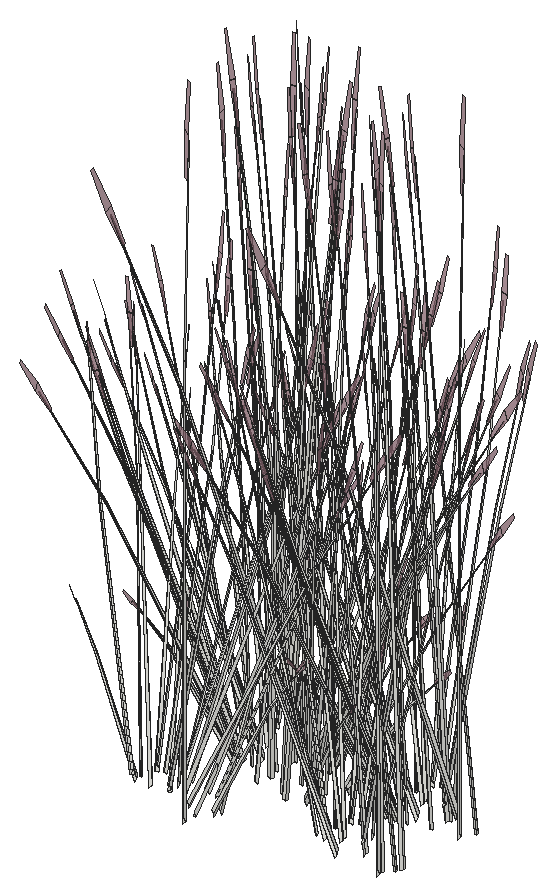
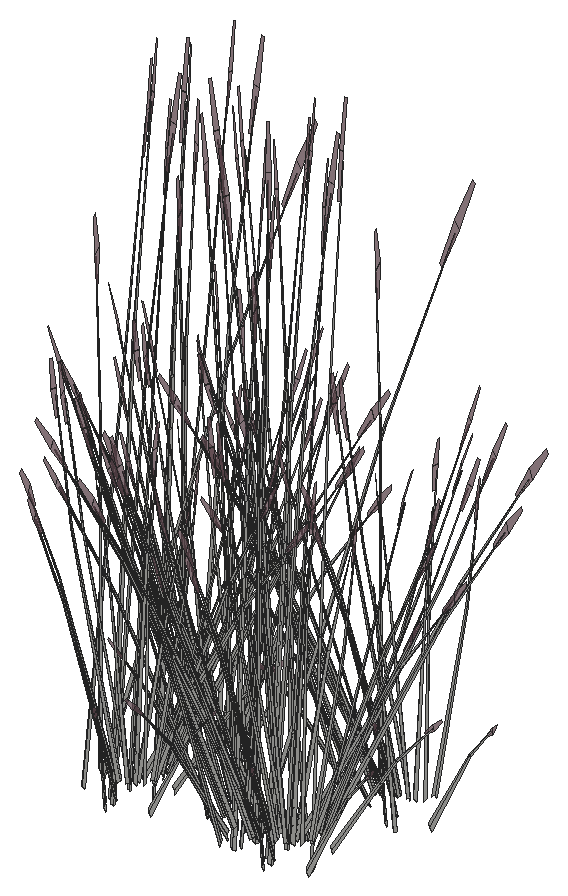
# SketchUp Ruby script. Lengths in inches.
U = 1.inch
M = Sketchup.active_model
def pt(a) = Geom::Point3d.new(a.map { |v| v * U })
def face(e, loops, mat)
  f = e.add_face(loops[0].map { |a| pt(a) })
  loops[1..].each { |l| e.add_face(l.map { |a| pt(a) }).erase! }
  f.material = f.back_material = mat if mat
  f
end
# faces: each face lists its corners as indices into pts; further lists are holes
def faces(e, pts, list, mat = nil) = list.each { |f| face(e, (f[0].is_a?(Array) ? f : [f]).map { |l| l.map { |i| pts[i] } }, mat) }
# xy, xz, yz: faces in a plane at the given z, y or x. An outline is a flat list of corners, or four numbers for a rectangle; further outlines are holes
def ring(l) = l.size == 4 ? [[l[0], l[1]], [l[2], l[1]], [l[2], l[3]], [l[0], l[3]]] : l.each_slice(2).to_a
def flat(e, list, mat, &to3) = list.each { |f| face(e, (f[0].is_a?(Array) ? f : [f]).map { |l| ring(l).map { |u, v| to3.(u, v) } }, mat) }
def xy(e, z, list, mat = nil) = flat(e, list, mat) { |x, y| [x, y, z] }
def xz(e, y, list, mat = nil) = flat(e, list, mat) { |x, z| [x, y, z] }
def yz(e, x, list, mat = nil) = flat(e, list, mat) { |y, z| [x, y, z] }
def lines(e, pts, list) = list.each { |a, b| e.add_line(pt(pts[a]), pt(pts[b])) }
# prism: a flat outline (further loops are holes) pulled along v
def prism(e, loops, v, mat = nil)
  f = face(e, loops, mat); d = Geom::Vector3d.new(v.map { |x| x * U })
  f.pushpull(f.normal.samedirection?(d) ? d.length : -d.length)
end
def box(e, o, s, mat = nil) = prism(e, [[o, [o[0] + s[0], o[1], o[2]], [o[0] + s[0], o[1] + s[1], o[2]], [o[0], o[1] + s[1], o[2]]]], [0, 0, s[2]], mat)
def at(x, y, z, deg = 0) = Geom::Transformation.translation(pt([x, y, z])) * Geom::Transformation.rotation(ORIGIN, Z_AXIS, deg.degrees)
def axes(o, x, y, z) = Geom::Transformation.new([*x, 0, *y, 0, *z, 0, *pt(o).to_a, 1])
def part(name) = M.definitions.add(name)
# library, detail: a bought-in or finely detailed component or shape, given as its bounding box
def library(name, o, s) = part(name).tap { |d| box(d.entities, o, s) }
def detail(e, o, s) = box(e.add_group.entities, o, s)
def put(e, d, t, mat = nil) = e.add_instance(d, t).tap { |i| i.material = mat if mat }
def group(e, t, mat = nil) = e.add_group.tap { |g| g.transformation = t; g.material = mat if mat }.entities
root = M.entities
M.materials.add("LightPink_Translucent").color = [144, 107, 117]
M.materials["LightPink_Translucent"].alpha = 0.75
c1 = part("blade")
p = [[2.15,0.21,22],[0,0.17,0],[0.09,0.45,0],[2.18,0.31,22],[2.29,0.31,22],[0.38,0.45,0],
  [2.48,0.24,33],[2.49,0.24,33],[2.48,0.22,33]]
faces(c1.entities,p,[[0,1,2,3],[4,5,2,3],[6,3,4,7],[8,0,3,6]])
c2 = part("seeds")
p = [[0.3,-0.1,1.38],[-0.01,-0.03,1.59],[-0.01,-0.03,0.03],[0.14,-0.07,-0.07],[0.29,-0.03,3],[0.15,0.01,3.11]]
faces(c2.entities,p,[[0,1,2,3],[1,0,4,5]],"LightPink_Translucent")
c3 = part("blade with seeds")
put(c3.entities,c1,at(0,0,0))
put(c3.entities,c2,axes([2.4,0.25,30.99],[1.5799,-0.05474,1.17369],[-0.12525,1.92788,0.29478],[-0.07173,-0.02425,1.56792]))
put(root,c3,axes([679.34,344.25,512.05],[0.18794,-0.56744,0.14643],[0.68774,0.16058,0.29122],[-0.1188,0.00276,1.33138]))
put(root,c3,axes([677.89,346.63,513.76],[-0.10048,-0.4599,-0.29394],[0.5744,-0.12144,0.37948],[-0.15428,-0.13179,0.72609]))
put(root,c3,axes([661.52,342.6,512.3],[0.27113,-0.25877,0.95334],[0.10699,0.40966,0.70045],[-0.19594,0.07335,0.20998]))
put(root,c3,axes([668.04,342.12,513.76],[0.37017,0.35748,-0.29394],[-0.42268,0.3384,0.37948],[0.21476,0.05149,0.72609]))
put(root,c3,axes([676.6,342.27,512.77],[0.18493,-0.0826,1.46963],[0.06377,0.5767,0.11501],[-0.40056,0.07652,0.52526]))
put(root,c3,axes([662.54,341.48,513.76],[-0.56631,0.0816,-0.29394],[-0.14954,-0.46647,0.37948],[-0.16229,0.12529,0.72609]))
put(root,c3,axes([677.03,344.51,512.06],[0.60889,0.28548,0.4121],[-0.36394,0.51192,0],[-0.13868,-0.06502,1.30728]))
put(root,c3,axes([665.35,347.1,513.22],[0.24166,0.09837,1.42242],[-0.50011,0.41269,0.11501],[-0.3117,-0.18617,0.60807]))
put(root,c3,axes([676.66,347.3,513.22],[0.24166,0.09837,1.42242],[-0.50011,0.41269,0.11501],[-0.3117,-0.18617,0.60807]))
put(root,c3,axes([675.33,342.59,513.89],[-0.17625,0.51936,-0.42412],[-0.60429,-0.17802,-0.32852],[-0.2433,0.04762,0.81151]))
put(root,c3,axes([666.52,346.81,513.89],[-0.64198,0.13573,-0.42412],[-0.1123,-0.514,-0.32852],[-0.17243,-0.1473,0.81151]))
put(root,c3,axes([666.71,341.2,513.22],[-0.24166,-0.09837,1.42242],[0.50011,-0.41269,0.11501],[0.3117,0.18617,0.60807]))
put(root,c3,axes([679.01,343.25,512.26],[0.70648,-0.03525,0.37133],[0.06389,0.58508,-0.17871],[-0.12647,0.0593,1.19224]))
put(root,c3,axes([677.82,347.01,513.89],[-0.64198,0.13573,-0.42412],[-0.1123,-0.514,-0.32852],[-0.17243,-0.1473,0.81151]))
put(root,c3,axes([670.31,348.03,514.13],[0.33983,-0.45051,-0.58968],[0.59551,0.32017,0.07116],[0.20291,-0.16322,0.83415]))
put(root,c3,axes([670.29,347.82,513.89],[-0.16713,-0.52135,-0.42412],[0.63294,-0.0912,-0.32852],[0.18138,-0.14003,0.81151]))
put(root,c3,axes([667.61,342.32,512.3],[-0.36631,-0.16417,0.95334],[0.47299,-0.16681,0.70045],[0.12758,0.1413,0.20998]))
put(root,c3,axes([663.01,341.53,513.89],[0.16713,0.52135,-0.42412],[-0.63294,0.0912,-0.32852],[-0.18138,0.14003,0.81151]))
put(root,c3,axes([668.1,349.91,512.76],[0.56221,0.23024,1.25546],[-0.55078,0.49601,0.49647],[-0.2467,-0.29398,1.05249]))
put(root,c3,axes([666.72,340.47,512.36],[-0.01777,-0.53759,1.17256],[0.80434,0.13935,0.49647],[-0.19024,0.29416,1.1068]))
put(root,c3,axes([675.31,342.85,513.22],[0.22574,-0.12077,1.42242],[0.19004,0.55807,0.11501],[-0.35439,0.12613,0.60807]))
put(root,c3,axes([666.78,342.55,513.89],[0.64198,-0.13573,-0.42412],[0.1123,0.514,-0.32852],[0.17243,0.1473,0.81151]))
put(root,c3,axes([679.41,350.12,512.76],[0.56221,0.23024,1.25546],[-0.55078,0.49601,0.49647],[-0.2467,-0.29398,1.05249]))
put(root,c3,axes([671.07,346.79,512.3],[-0.2167,0.29065,0.95334],[-0.18626,-0.3905,0.70045],[0.17898,-0.09785,0.20998]))
put(root,c3,axes([667.67,343.07,512.21],[-0.4172,-0.01791,0.872],[0.27552,-0.38032,0.48145],[0.16481,0.13512,0.68401]))
put(root,c3,axes([679.53,344.55,512.06],[0.60889,-0.28548,0.4121],[0.36394,0.51192,0],[-0.13868,0.06502,1.30728]))
put(root,c3,axes([670.76,347.88,513.76],[0.56631,-0.0816,-0.29394],[0.14954,0.46647,0.37948],[0.16229,-0.12529,0.72609]))
put(root,c3,axes([665.25,347.24,513.76],[-0.37017,-0.35748,-0.29394],[0.42268,-0.3384,0.37948],[-0.21476,-0.05149,0.72609]))
put(root,c3,axes([663.4,341.45,513.22],[0.12114,-0.19625,1.42242],[0.50818,0.40613,0.11501],[-0.22925,0.25313,0.60807]))
put(root,c3,axes([674.13,344.81,512.3],[0.27113,-0.25877,0.95334],[0.10699,0.40966,0.70045],[-0.19594,0.07335,0.20998]))
put(root,c3,axes([676.5625,347.44,513.76],[-0.37017,-0.35748,-0.29394],[0.42268,-0.3384,0.37948],[-0.21476,-0.05149,0.72609]))
put(root,c3,axes([666.31,342.15,512.15],[0.01148,-0.18927,1.18691],[0.54864,-0.21141,-0.25526],[0.16937,0.22654,0.50747]))
put(root,c3,axes([675.15,343.6875,513.76],[-0.56631,0.0816,-0.29394],[-0.14954,-0.46647,0.37948],[-0.16229,0.12529,0.72609]))
put(root,c3,axes([663.54,342.56,513.76],[-0.4402,0.30062,-0.29394],[-0.41671,-0.34326,0.37948],[-0.0634,0.1744,0.72609]))
put(root,c3,axes([663.82,343.72,512.3],[-0.01684,-0.3395,0.95334],[0.42072,0.24214,0.70045],[-0.08274,0.16182,0.20998]))
put(root,c3,axes([665.64,347.47,514.13],[-0.65035,-0.01375,-0.58968],[0.04368,-0.5789,0.07116],[-0.27552,-0.06109,0.83415]))
put(root,c3,axes([676.95,347.68,514.13],[-0.65035,-0.01375,-0.58968],[0.04368,-0.5789,0.07116],[-0.27552,-0.06109,0.83415]))
put(root,c3,axes([663.97,342.41,514.15],[0.46573,0.38364,-0.47077],[-0.49199,0.33598,-0.36465],[-0.07086,0.19492,0.90078]))
put(root,c3,axes([665.36,342.79,513.89],[0.63954,0.14313,-0.42412],[-0.21921,0.49074,-0.32852],[0.05864,0.19758,0.81151]))
put(root,c3,axes([665.72,341.77,513.22],[-0.14872,-0.18332,1.42242],[0.6872,-0.15433,0.11501],[0.15531,0.28779,0.60807]))
put(root,c3,axes([665.0625,343.09,513.76],[-0.19614,0.43908,-0.29394],[-0.57222,-0.12807,0.37948],[0.05247,0.17678,0.72609]))
put(root,c3,axes([676.13,343.23,513.22],[0.1625,-0.17544,1.42242],[0.41029,0.47354,0.11501],[-0.28141,0.21565,0.60807]))
put(root,c3,axes([665.43,347.59,513.89],[-0.47241,0.37822,-0.42412],[-0.41372,-0.39954,-0.32852],[-0.24002,-0.05755,0.81151]))
put(root,c3,axes([663.83,342.24,514.43],[-0.01693,0.52814,-0.65454],[-0.71285,-0.03547,0.07899],[-0.07523,0.22375,0.92591]))
put(root,c3,axes([675.62,343.74,513.89],[0.16713,0.52135,-0.42412],[-0.63294,0.0912,-0.32852],[-0.18138,0.14003,0.81151]))
put(root,c3,axes([664.36,348.09,512.3],[0.41536,-0.04086,0.95334],[-0.26347,0.35999,0.70045],[-0.20525,-0.054,0.20998]))
put(root,c3,axes([676.74,347.8,513.89],[-0.47241,0.37822,-0.42412],[-0.41372,-0.39954,-0.32852],[-0.24002,-0.05755,0.81151]))
put(root,c3,axes([664.5,341.86,513.22],[-0.01592,-0.21915,1.42242],[0.69015,0.14538,0.11501],[-0.04269,0.3123,0.60807]))
put(root,c3,axes([679.33,342.6875,512.36],[-0.01777,-0.53759,1.17256],[0.80434,0.13935,0.49647],[-0.19024,0.29416,1.1068]))
put(root,c3,axes([667.3,348.43,512.26],[-0.70648,0.03525,0.37133],[-0.06389,-0.58508,-0.17871],[0.12647,-0.0593,1.19224]))
put(root,c3,axes([665.48,348.85,512.06],[0,0.57097,0.4121],[-0.72788,0,0],[0,-0.13004,1.30728]))
put(root,c3,axes([675.67,348.3,512.3],[0.41536,-0.04086,0.95334],[-0.26347,0.35999,0.70045],[-0.20525,-0.054,0.20998]))
put(root,c3,axes([670.58,348.98,513.89],[0.17625,-0.51936,-0.42412],[0.60429,0.17802,-0.32852],[0.2433,-0.04762,0.81151]))
put(root,c3,axes([664.84,348,513.22],[0.26985,-0.01293,1.42242],[-0.17902,0.56047,0.11501],[-0.38456,-0.03467,0.60807]))
put(root,c3,axes([665.125,342.69,514.13],[0.31051,0.46426,-0.58968],[-0.63919,0.25873,0.07116],[0.07261,0.22432,0.83415]))
put(root,c3,axes([676.78,349.06,512.06],[0,0.57097,0.4121],[-0.72788,0,0],[0,-0.13004,1.30728]))
put(root,c3,axes([663.33,343.42,512.15],[0.2053,-0.09007,1.18691],[0.50689,0.27159,-0.25526],[-0.15087,0.235,0.50747]))
put(root,c3,axes([676.15,348.2,513.22],[0.26985,-0.01293,1.42242],[-0.17902,0.56047,0.11501],[-0.38456,-0.03467,0.60807]))
put(root,c3,axes([667.13,349.14,512.26],[-0.31565,0.51449,0.37133],[-0.65588,-0.24761,-0.17871],[0,-0.1186,1.19224]))
put(root,c3,axes([669.28,347.16,512.06],[-0.60889,-0.28548,0.4121],[0.36394,-0.51192,0],[0.13868,0.06502,1.30728]))
put(root,c3,axes([670.47,349.17,514.13],[0.57168,-0.25217,-0.58968],[0.3186,0.51908,0.07116],[0.27622,-0.05897,0.83415]))
put(root,c3,axes([678.44,349.34,512.26],[-0.31565,0.51449,0.37133],[-0.65588,-0.24761,-0.17871],[0,-0.1186,1.19224]))
put(root,c3,axes([676.01,343.66,513.22],[0.12114,-0.19625,1.42242],[0.50818,0.40613,0.11501],[-0.22925,0.25313,0.60807]))
put(root,c3,axes([666.97,347.42,512.05],[-0.18794,0.56744,0.14643],[-0.68774,-0.16058,0.29122],[0.1188,-0.00276,1.33138]))
put(root,c3,axes([663.59,342.98,512.79],[0.01429,-0.29475,1.28107],[0.64291,0.15569,0.17703],[-0.0557,0.31414,0.60492]))
put(root,c3,axes([676.15,344.77,513.76],[-0.4402,0.30062,-0.29394],[-0.41671,-0.34326,0.37948],[-0.0634,0.1744,0.72609]))
put(root,c3,axes([676.43,345.9375,512.3],[-0.01684,-0.3395,0.95334],[0.42072,0.24214,0.70045],[-0.08274,0.16182,0.20998]))
put(root,c3,axes([668.14,348.1875,512.26],[-0.39083,-0.47924,0.37133],[0.59199,-0.33747,-0.17871],[0.12647,0.0593,1.19224]))
put(root,c3,axes([666.9,350.35,512.05],[0.6991,-0.15154,0.14643],[0.17263,0.56398,0.29122],[-0.06235,-0.08217,1.33138]))
put(root,c3,axes([670.95,349.22,513.76],[0.54068,0.15928,-0.29394],[-0.1577,0.46469,0.37948],[0.21769,-0.04261,0.72609]))
put(root,c3,axes([676.59,344.625,514.15],[0.46573,0.38364,-0.47077],[-0.49199,0.33598,-0.36465],[-0.07086,0.19492,0.90078]))
put(root,c3,axes([664.6,348.48,513.76],[-0.54068,-0.15928,-0.29394],[0.1577,-0.46469,0.37948],[-0.21769,0.04261,0.72609]))
put(root,c3,axes([678.21,350.55,512.05],[0.6991,-0.15154,0.14643],[0.17263,0.56398,0.29122],[-0.06235,-0.08217,1.33138]))
put(root,c3,axes([669.05,347.45,512.05],[-0.6991,0.15154,0.14643],[-0.17263,-0.56398,0.29122],[0.06235,0.08217,1.33138]))
put(root,c3,axes([677.68,345.3,513.76],[-0.19614,0.43908,-0.29394],[-0.57222,-0.12807,0.37948],[0.05247,0.17678,0.72609]))
put(root,c3,axes([675.91,348.68,513.76],[-0.54068,-0.15928,-0.29394],[0.1577,-0.46469,0.37948],[-0.21769,0.04261,0.72609]))
put(root,c3,axes([669.48,348.64,513.22],[-0.26985,0.01293,1.42242],[0.17902,-0.56047,0.11501],[0.38456,0.03467,0.60807]))
put(root,c3,axes([676.44,344.45,514.43],[-0.01693,0.52814,-0.65454],[-0.71285,-0.03547,0.07899],[-0.07523,0.22375,0.92591]))
put(root,c3,axes([677.12,344.08,513.22],[-0.01592,-0.21915,1.42242],[0.69015,0.14538,0.11501],[-0.04269,0.3123,0.60807]))
put(root,c3,axes([668.98,350.38,512.05],[0.18794,-0.56744,0.14643],[0.68774,0.16058,0.29122],[-0.1188,0.00276,1.33138]))
put(root,c3,axes([666.25,348.4,512.77],[0.18493,-0.0826,1.46963],[0.06377,0.5767,0.11501],[-0.40056,0.07652,0.52526]))
put(root,c3,axes([670.06,348.93,512.05],[-0.51116,-0.4159,0.14643],[0.51512,-0.4034,0.29122],[-0.05645,0.08494,1.33138]))
put(root,c3,axes([680.29,350.58,512.05],[0.18794,-0.56744,0.14643],[0.68774,0.16058,0.29122],[-0.1188,0.00276,1.33138]))
put(root,c3,axes([672.1,349.3125,512.3],[-0.40197,0.09426,0.95334],[0.18921,-0.38956,0.70045],[0.21325,0.02666,0.20998]))
put(root,c3,axes([666.68,350.64,512.06],[0.60889,0.28548,0.4121],[-0.36394,0.51192,0],[-0.13868,-0.06502,1.30728]))
put(root,c3,axes([677.55,348.6,512.77],[0.18493,-0.0826,1.46963],[0.06377,0.5767,0.11501],[-0.40056,0.07652,0.52526]))
put(root,c3,axes([668.82,348.66,512.26],[0.31565,-0.51449,0.37133],[0.65588,0.24761,-0.17871],[0,0.1186,1.19224]))
put(root,c3,axes([677.98,350.84,512.06],[0.60889,0.28548,0.4121],[-0.36394,0.51192,0],[-0.13868,-0.06502,1.30728]))
put(root,c3,axes([664.97,348.71,513.89],[-0.17625,0.51936,-0.42412],[-0.60429,-0.17802,-0.32852],[-0.2433,0.04762,0.81151]))
put(root,c3,axes([671.4,350.51,513.26],[-0.12452,-0.47997,-0.02898],[0.58854,-0.11034,-0.1314],[0.1229,0.03043,0.43341]))
put(root,c3,axes([670.48,348.95,512.06],[0,-0.57097,0.4121],[0.72788,0,0],[0,0.13004,1.30728]))
put(root,c3,axes([676.21,345.19,512.79],[0.01429,-0.29475,1.28107],[0.64291,0.15569,0.17703],[-0.0557,0.31414,0.60492]))
put(root,c3,axes([676.28,348.92,513.89],[-0.17625,0.51936,-0.42412],[-0.60429,-0.17802,-0.32852],[-0.2433,0.04762,0.81151]))
put(root,c3,axes([668.65,349.375,512.26],[0.70648,-0.03525,0.37133],[0.06389,0.58508,-0.17871],[-0.12647,0.0593,1.19224]))
put(root,c3,axes([671.35,349.9375,512.15],[-0.15668,-0.14043,1.18691],[0.20386,-0.46454,-0.25526],[0.31701,0.06293,0.50747]))
put(root,c3,axes([664.95,348.98,513.22],[0.22574,-0.12077,1.42242],[0.19004,0.55807,0.11501],[-0.35439,0.12613,0.60807]))
put(root,c3,axes([676.26,349.19,513.22],[0.22574,-0.12077,1.42242],[0.19004,0.55807,0.11501],[-0.35439,0.12613,0.60807]))
put(root,c3,axes([669.91,350.22,514.13],[0.65035,0.01375,-0.58968],[-0.04368,0.5789,0.07116],[0.27552,0.06109,0.83415]))
put(root,c3,axes([669.18,350.68,512.06],[0.60889,-0.28548,0.4121],[0.36394,0.51192,0],[-0.13868,0.06502,1.30728]))
put(root,c3,axes([664.25,349.93,512.15],[0.2261,0.04687,1.18691],[0.14573,0.47875,-0.25526],[-0.30712,0.08962,0.50747]))
put(root,c3,axes([663.77,350.9375,512.3],[0.27113,-0.25877,0.95334],[0.10699,0.40966,0.70045],[-0.19594,0.07335,0.20998]))
put(root,c3,axes([670.3,350.46,513.76],[0.37017,0.35748,-0.29394],[-0.42268,0.3384,0.37948],[0.21476,0.05149,0.72609]))
put(root,c3,axes([664.8,349.82,513.76],[-0.56631,0.0816,-0.29394],[-0.14954,-0.46647,0.37948],[-0.16229,0.12529,0.72609]))
put(root,c3,axes([675.08,351.14,512.3],[0.27113,-0.25877,0.95334],[0.10699,0.40966,0.70045],[-0.19594,0.07335,0.20998]))
put(root,c3,axes([676.11,350.02,513.76],[-0.56631,0.0816,-0.29394],[-0.14954,-0.46647,0.37948],[-0.16229,0.12529,0.72609]))
put(root,c3,axes([668.97,349.54,513.22],[-0.24166,-0.09837,1.42242],[0.50011,-0.41269,0.11501],[0.3117,0.18617,0.60807]))
put(root,c3,axes([669.87,350.66,512.3],[-0.36631,-0.16417,0.95334],[0.47299,-0.16681,0.70045],[0.12758,0.1413,0.20998]))
put(root,c3,axes([665.78,349.36,513.22],[0.1625,-0.17544,1.42242],[0.41029,0.47354,0.11501],[-0.28141,0.21565,0.60807]))
put(root,c3,axes([665.26,349.87,513.89],[0.16713,0.52135,-0.42412],[-0.63294,0.0912,-0.32852],[-0.18138,0.14003,0.81151]))
put(root,c3,axes([677.08,349.5625,513.22],[0.1625,-0.17544,1.42242],[0.41029,0.47354,0.11501],[-0.28141,0.21565,0.60807]))
put(root,c3,axes([676.57,350.07,513.89],[0.16713,0.52135,-0.42412],[-0.63294,0.0912,-0.32852],[-0.18138,0.14003,0.81151]))
put(root,c3,axes([668.97,348.81,512.36],[-0.01777,-0.53759,1.17256],[0.80434,0.13935,0.49647],[-0.19024,0.29416,1.1068]))
put(root,c3,axes([669.04,350.89,513.89],[0.64198,-0.13573,-0.42412],[0.1123,0.514,-0.32852],[0.17243,0.1473,0.81151]))
put(root,c3,axes([680.28,349.02,512.36],[-0.01777,-0.53759,1.17256],[0.80434,0.13935,0.49647],[-0.19024,0.29416,1.1068]))
put(root,c3,axes([669.92,351.41,512.21],[-0.4172,-0.01791,0.872],[0.27552,-0.38032,0.48145],[0.16481,0.13512,0.68401]))
put(root,c3,axes([665.65,349.79,513.22],[0.12114,-0.19625,1.42242],[0.50818,0.40613,0.11501],[-0.22925,0.25313,0.60807]))
put(root,c3,axes([676.96,349.99,513.22],[0.12114,-0.19625,1.42242],[0.50818,0.40613,0.11501],[-0.22925,0.25313,0.60807]))
put(root,c3,axes([665.79,350.9,513.76],[-0.4402,0.30062,-0.29394],[-0.41671,-0.34326,0.37948],[-0.0634,0.1744,0.72609]))
put(root,c3,axes([666.07,352.06,512.3],[-0.01684,-0.3395,0.95334],[0.42072,0.24214,0.70045],[-0.08274,0.16182,0.20998]))
put(root,c3,axes([677.1,351.1,513.76],[-0.4402,0.30062,-0.29394],[-0.41671,-0.34326,0.37948],[-0.0634,0.1744,0.72609]))
put(root,c3,axes([677.38,352.27,512.3],[-0.01684,-0.3395,0.95334],[0.42072,0.24214,0.70045],[-0.08274,0.16182,0.20998]))
put(root,c3,axes([666.23,350.75,514.15],[0.46573,0.38364,-0.47077],[-0.49199,0.33598,-0.36465],[-0.07086,0.19492,0.90078]))
put(root,c3,axes([667.61,351.125,513.89],[0.63954,0.14313,-0.42412],[-0.21921,0.49074,-0.32852],[0.05864,0.19758,0.81151]))
put(root,c3,axes([667.98,350.11,513.22],[-0.14872,-0.18332,1.42242],[0.6872,-0.15433,0.11501],[0.15531,0.28779,0.60807]))
put(root,c3,axes([677.54,350.96,514.15],[0.46573,0.38364,-0.47077],[-0.49199,0.33598,-0.36465],[-0.07086,0.19492,0.90078]))
put(root,c3,axes([667.32,351.43,513.76],[-0.19614,0.43908,-0.29394],[-0.57222,-0.12807,0.37948],[0.05247,0.17678,0.72609]))
put(root,c3,axes([666.09,350.58,514.43],[-0.01693,0.52814,-0.65454],[-0.71285,-0.03547,0.07899],[-0.07523,0.22375,0.92591]))
put(root,c3,axes([666.76,350.2,513.22],[-0.01592,-0.21915,1.42242],[0.69015,0.14538,0.11501],[-0.04269,0.3123,0.60807]))
put(root,c3,axes([677.4,350.78,514.43],[-0.01693,0.52814,-0.65454],[-0.71285,-0.03547,0.07899],[-0.07523,0.22375,0.92591]))
put(root,c3,axes([678.07,350.41,513.22],[-0.01592,-0.21915,1.42242],[0.69015,0.14538,0.11501],[-0.04269,0.3123,0.60807]))
put(root,c3,axes([667.38,351.03,514.13],[0.31051,0.46426,-0.58968],[-0.63919,0.25873,0.07116],[0.07261,0.22432,0.83415]))
put(root,c3,axes([665.85,351.32,512.79],[0.01429,-0.29475,1.28107],[0.64291,0.15569,0.17703],[-0.0557,0.31414,0.60492]))
put(root,c3,axes([677.16,351.53,512.79],[0.01429,-0.29475,1.28107],[0.64291,0.15569,0.17703],[-0.0557,0.31414,0.60492]))
